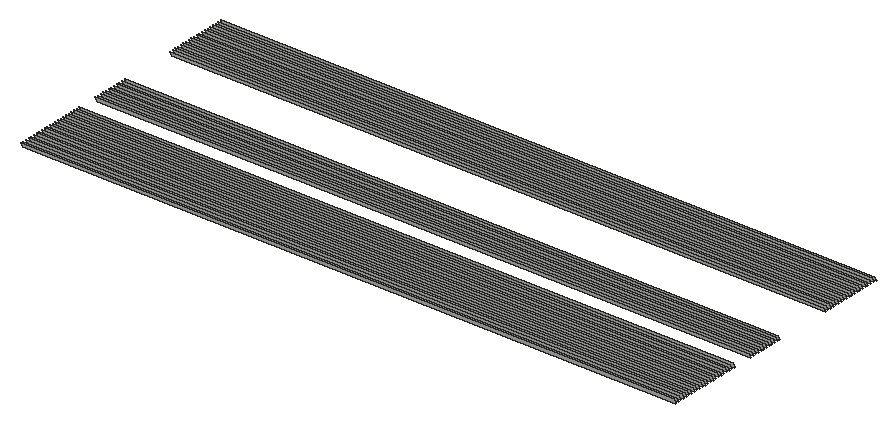
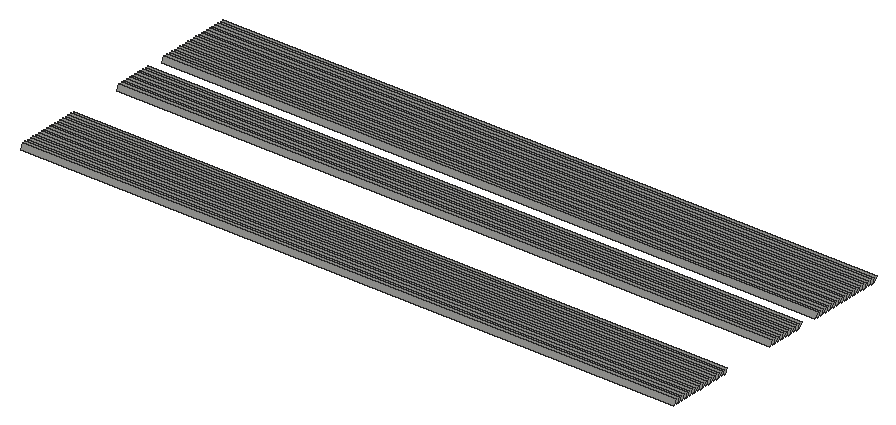
# SketchUp Ruby script. Lengths in inches.
U = 1.inch
M = Sketchup.active_model
def pt(a) = Geom::Point3d.new(a.map { |v| v * U })
def face(e, loops, mat)
  f = e.add_face(loops[0].map { |a| pt(a) })
  loops[1..].each { |l| e.add_face(l.map { |a| pt(a) }).erase! }
  f.material = f.back_material = mat if mat
  f
end
# faces: each face lists its corners as indices into pts; further lists are holes
def faces(e, pts, list, mat = nil) = list.each { |f| face(e, (f[0].is_a?(Array) ? f : [f]).map { |l| l.map { |i| pts[i] } }, mat) }
# xy, xz, yz: faces in a plane at the given z, y or x. An outline is a flat list of corners, or four numbers for a rectangle; further outlines are holes
def ring(l) = l.size == 4 ? [[l[0], l[1]], [l[2], l[1]], [l[2], l[3]], [l[0], l[3]]] : l.each_slice(2).to_a
def flat(e, list, mat, &to3) = list.each { |f| face(e, (f[0].is_a?(Array) ? f : [f]).map { |l| ring(l).map { |u, v| to3.(u, v) } }, mat) }
def xy(e, z, list, mat = nil) = flat(e, list, mat) { |x, y| [x, y, z] }
def xz(e, y, list, mat = nil) = flat(e, list, mat) { |x, z| [x, y, z] }
def yz(e, x, list, mat = nil) = flat(e, list, mat) { |y, z| [x, y, z] }
def lines(e, pts, list) = list.each { |a, b| e.add_line(pt(pts[a]), pt(pts[b])) }
# prism: a flat outline (further loops are holes) pulled along v
def prism(e, loops, v, mat = nil)
  f = face(e, loops, mat); d = Geom::Vector3d.new(v.map { |x| x * U })
  f.pushpull(f.normal.samedirection?(d) ? d.length : -d.length)
end
def box(e, o, s, mat = nil) = prism(e, [[o, [o[0] + s[0], o[1], o[2]], [o[0] + s[0], o[1] + s[1], o[2]], [o[0], o[1] + s[1], o[2]]]], [0, 0, s[2]], mat)
def at(x, y, z, deg = 0) = Geom::Transformation.translation(pt([x, y, z])) * Geom::Transformation.rotation(ORIGIN, Z_AXIS, deg.degrees)
def axes(o, x, y, z) = Geom::Transformation.new([*x, 0, *y, 0, *z, 0, *pt(o).to_a, 1])
def part(name) = M.definitions.add(name)
# library, detail: a bought-in or finely detailed component or shape, given as its bounding box
def library(name, o, s) = part(name).tap { |d| box(d.entities, o, s) }
def detail(e, o, s) = box(e.add_group.entities, o, s)
def put(e, d, t, mat = nil) = e.add_instance(d, t).tap { |i| i.material = mat if mat }
def group(e, t, mat = nil) = e.add_group.tap { |g| g.transformation = t; g.material = mat if mat }.entities
root = M.entities
c1 = part("Group133\#1")
p = [[385.16,-531.55,0],[-385.16,-531.55,0],[-385.16,-534.9375,5.875],[385.16,-534.9375,5.875]]
faces(c1.entities,p,[[0,1,2,3]])
c2 = part("Group134\#1")
p = [[385.16,-527.61,0],[-385.16,-527.61,0],[-385.16,-531,5.875],[385.16,-531,5.875]]
faces(c2.entities,p,[[0,1,2,3]])
c3 = part("Group135\#1")
p = [[-385.16,-527.0625,5.875],[385.16,-527.0625,5.875],[385.16,-523.67,0],[-385.16,-523.67,0]]
faces(c3.entities,p,[[0,1,2,3]])
c4 = part("Group136\#1")
p = [[-385.16,-523.125,5.875],[385.16,-523.125,5.875],[385.16,-519.73,0],[-385.16,-519.73,0]]
faces(c4.entities,p,[[0,1,2,3]])
c5 = part("Group137\#1")
p = [[-385.16,-519.1875,5.875],[385.16,-519.1875,5.875],[385.16,-515.8,0],[-385.16,-515.8,0]]
faces(c5.entities,p,[[0,1,2,3]])
c6 = part("Group138\#1")
p = [[-385.16,-515.25,5.875],[385.16,-515.25,5.875],[385.16,-511.86,0],[-385.16,-511.86,0]]
faces(c6.entities,p,[[0,1,2,3]])
c7 = part("Group139\#1")
p = [[385.16,-507.92,0],[-385.16,-507.92,0],[-385.16,-511.3125,5.875],[385.16,-511.3125,5.875]]
faces(c7.entities,p,[[0,1,2,3]])
c8 = part("Group140\#1")
p = [[385.16,-503.98,0],[-385.16,-503.98,0],[-385.16,-507.375,5.875],[385.16,-507.375,5.875]]
faces(c8.entities,p,[[0,1,2,3]])
c9 = part("Group141\#1")
p = [[-385.16,-503.4375,5.875],[385.16,-503.4375,5.875],[385.16,-500.05,0],[-385.16,-500.05,0]]
faces(c9.entities,p,[[0,1,2,3]])
c10 = part("Group142\#1")
p = [[-385.16,-499.5,5.875],[385.16,-499.5,5.875],[385.16,-496.11,0],[-385.16,-496.11,0]]
faces(c10.entities,p,[[0,1,2,3]])
c11 = part("Group143\#1")
p = [[-385.16,-495.5625,5.875],[385.16,-495.5625,5.875],[385.16,-492.17,0],[-385.16,-492.17,0]]
faces(c11.entities,p,[[0,1,2,3]])
c12 = part("Group144\#1")
p = [[-385.16,-491.625,5.875],[385.16,-491.625,5.875],[385.16,-488.23,0],[-385.16,-488.23,0]]
faces(c12.entities,p,[[0,1,2,3]])
c13 = part("Group145\#1")
p = [[-385.16,-487.6875,5.875],[385.16,-487.6875,5.875],[385.16,-484.3,0],[-385.16,-484.3,0]]
faces(c13.entities,p,[[0,1,2,3]])
c14 = part("Group146\#1")
p = [[385.16,-480.36,0],[-385.16,-480.36,0],[-385.16,-483.75,5.875],[385.16,-483.75,5.875]]
faces(c14.entities,p,[[0,1,2,3]])
c15 = part("Group147\#1")
p = [[-385.16,-479.8125,5.875],[385.16,-479.8125,5.875],[385.16,-476.42,0],[-385.16,-476.42,0]]
faces(c15.entities,p,[[0,1,2,3]])
c16 = part("Group148\#1")
p = [[385.16,-472.48,0],[-385.16,-472.48,0],[-385.16,-475.875,5.875],[385.16,-475.875,5.875]]
faces(c16.entities,p,[[0,1,2,3]])
c17 = part("Group149\#1")
p = [[-385.16,-471.9375,5.875],[385.16,-471.9375,5.875],[385.16,-468.55,0],[-385.16,-468.55,0]]
faces(c17.entities,p,[[0,1,2,3]])
c18 = part("Group150\#1")
p = [[-385.16,-468,5.875],[385.16,-468,5.875],[385.16,-464.61,0],[-385.16,-464.61,0]]
faces(c18.entities,p,[[0,1,2,3]])
c19 = part("Group151\#1")
p = [[-385.16,-464.0625,5.875],[385.16,-464.0625,5.875],[385.16,-460.67,0],[-385.16,-460.67,0]]
faces(c19.entities,p,[[0,1,2,3]])
c20 = part("Group152\#1")
p = [[-385.16,-460.125,5.875],[385.16,-460.125,5.875],[385.16,-456.73,0],[-385.16,-456.73,0]]
faces(c20.entities,p,[[0,1,2,3]])
c21 = part("Group153\#1")
p = [[385.16,-452.8,0],[-385.16,-452.8,0],[-385.16,-456.1875,5.875],[385.16,-456.1875,5.875]]
faces(c21.entities,p,[[0,1,2,3]])
c22 = part("Group154\#1")
p = [[-385.16,-452.25,5.875],[385.16,-452.25,5.875],[385.16,-448.86,0],[-385.16,-448.86,0]]
faces(c22.entities,p,[[0,1,2,3]])
c23 = part("Group155\#1")
p = [[-385.16,-448.3125,5.875],[385.16,-448.3125,5.875],[385.16,-444.92,0],[-385.16,-444.92,0]]
faces(c23.entities,p,[[0,1,2,3]])
c24 = part("Group161\#1")
p = [[-385.16,-424.6875,5.875],[385.16,-424.6875,5.875],[385.16,-421.3,0],[-385.16,-421.3,0]]
faces(c24.entities,p,[[0,1,2,3]])
c25 = part("Group162\#1")
p = [[-385.16,-420.75,5.875],[385.16,-420.75,5.875],[385.16,-417.36,0],[-385.16,-417.36,0]]
faces(c25.entities,p,[[0,1,2,3]])
c26 = part("Group163\#1")
p = [[385.16,-413.42,0],[-385.16,-413.42,0],[-385.16,-416.8125,5.875],[385.16,-416.8125,5.875]]
faces(c26.entities,p,[[0,1,2,3]])
c27 = part("Group164\#1")
p = [[-385.16,-412.875,5.875],[385.16,-412.875,5.875],[385.16,-409.48,0],[-385.16,-409.48,0]]
faces(c27.entities,p,[[0,1,2,3]])
c28 = part("Group165\#1")
p = [[385.16,-405.55,0],[-385.16,-405.55,0],[-385.16,-408.9375,5.875],[385.16,-408.9375,5.875]]
faces(c28.entities,p,[[0,1,2,3]])
c29 = part("Group166\#1")
p = [[385.16,-401.61,0],[-385.16,-401.61,0],[-385.16,-405,5.875],[385.16,-405,5.875]]
faces(c29.entities,p,[[0,1,2,3]])
c30 = part("Group167\#1")
p = [[385.16,-397.67,0],[-385.16,-397.67,0],[-385.16,-401.0625,5.875],[385.16,-401.0625,5.875]]
faces(c30.entities,p,[[0,1,2,3]])
c31 = part("Group168\#1")
p = [[385.16,-393.73,0],[-385.16,-393.73,0],[-385.16,-397.125,5.875],[385.16,-397.125,5.875]]
faces(c31.entities,p,[[0,1,2,3]])
c32 = part("Group169\#1")
p = [[385.16,-389.8,0],[-385.16,-389.8,0],[-385.16,-393.1875,5.875],[385.16,-393.1875,5.875]]
faces(c32.entities,p,[[0,1,2,3]])
c33 = part("Group170\#1")
p = [[-385.16,-389.25,5.875],[385.16,-389.25,5.875],[385.16,-385.86,0],[-385.16,-385.86,0]]
faces(c33.entities,p,[[0,1,2,3]])
c34 = part("Group171\#1")
p = [[385.16,-381.92,0],[-385.16,-381.92,0],[-385.16,-385.3125,5.875],[385.16,-385.3125,5.875]]
faces(c34.entities,p,[[0,1,2,3]])
c35 = part("Group172\#1")
p = [[385.16,-377.98,0],[-385.16,-377.98,0],[-385.16,-381.375,5.875],[385.16,-381.375,5.875]]
faces(c35.entities,p,[[0,1,2,3]])
c36 = part("Group189\#1")
p = [[-385.16,-314.4375,5.875],[385.16,-314.4375,5.875],[385.16,-311.05,0],[-385.16,-311.05,0]]
faces(c36.entities,p,[[0,1,2,3]])
c37 = part("Group190\#1")
p = [[385.16,-307.11,0],[-385.16,-307.11,0],[-385.16,-310.5,5.875],[385.16,-310.5,5.875]]
faces(c37.entities,p,[[0,1,2,3]])
c38 = part("Group191\#1")
p = [[385.16,-303.17,0],[-385.16,-303.17,0],[-385.16,-306.5625,5.875],[385.16,-306.5625,5.875]]
faces(c38.entities,p,[[0,1,2,3]])
c39 = part("Group192\#1")
p = [[-385.16,-302.625,5.875],[385.16,-302.625,5.875],[385.16,-299.23,0],[-385.16,-299.23,0]]
faces(c39.entities,p,[[0,1,2,3]])
c40 = part("Group193\#1")
p = [[-385.16,-298.6875,5.875],[385.16,-298.6875,5.875],[385.16,-295.3,0],[-385.16,-295.3,0]]
faces(c40.entities,p,[[0,1,2,3]])
c41 = part("Group194\#1")
p = [[385.16,-291.36,0],[-385.16,-291.36,0],[-385.16,-294.75,5.875],[385.16,-294.75,5.875]]
faces(c41.entities,p,[[0,1,2,3]])
c42 = part("Group195\#1")
p = [[385.16,-287.42,0],[-385.16,-287.42,0],[-385.16,-290.8125,5.875],[385.16,-290.8125,5.875]]
faces(c42.entities,p,[[0,1,2,3]])
c43 = part("Group196\#1")
p = [[-385.16,-286.875,5.875],[385.16,-286.875,5.875],[385.16,-283.48,0],[-385.16,-283.48,0]]
faces(c43.entities,p,[[0,1,2,3]])
c44 = part("Group197\#1")
p = [[-385.16,-282.9375,5.875],[385.16,-282.9375,5.875],[385.16,-279.55,0],[-385.16,-279.55,0]]
faces(c44.entities,p,[[0,1,2,3]])
c45 = part("Group198\#1")
p = [[385.16,-275.61,0],[-385.16,-275.61,0],[-385.16,-279,5.875],[385.16,-279,5.875]]
faces(c45.entities,p,[[0,1,2,3]])
c46 = part("Group199\#1")
p = [[-385.16,-275.0625,5.875],[385.16,-275.0625,5.875],[385.16,-271.67,0],[-385.16,-271.67,0]]
faces(c46.entities,p,[[0,1,2,3]])
c47 = part("Group200\#1")
p = [[-385.16,-271.125,5.875],[385.16,-271.125,5.875],[385.16,-267.73,0],[-385.16,-267.73,0]]
faces(c47.entities,p,[[0,1,2,3]])
c48 = part("Group201\#1")
p = [[-385.16,-267.1875,5.875],[385.16,-267.1875,5.875],[385.16,-263.8,0],[-385.16,-263.8,0]]
faces(c48.entities,p,[[0,1,2,3]])
c49 = part("Group202\#1")
p = [[-385.16,-263.25,5.875],[385.16,-263.25,5.875],[385.16,-259.86,0],[-385.16,-259.86,0]]
faces(c49.entities,p,[[0,1,2,3]])
c50 = part("Group203\#1")
p = [[-385.16,-259.3125,5.875],[385.16,-259.3125,5.875],[385.16,-255.92,0],[-385.16,-255.92,0]]
faces(c50.entities,p,[[0,1,2,3]])
c51 = part("Group204\#1")
p = [[-385.16,-255.375,5.875],[385.16,-255.375,5.875],[385.16,-251.98,0],[-385.16,-251.98,0]]
faces(c51.entities,p,[[0,1,2,3]])
c52 = part("Group205\#1")
p = [[385.16,-248.05,0],[-385.16,-248.05,0],[-385.16,-251.4375,5.875],[385.16,-251.4375,5.875]]
faces(c52.entities,p,[[0,1,2,3]])
c53 = part("Group206\#1")
p = [[-385.16,-247.5,5.875],[385.16,-247.5,5.875],[385.16,-244.11,0],[-385.16,-244.11,0]]
faces(c53.entities,p,[[0,1,2,3]])
c54 = part("Group207\#1")
p = [[-385.16,-243.5625,5.875],[385.16,-243.5625,5.875],[385.16,-240.17,0],[-385.16,-240.17,0]]
faces(c54.entities,p,[[0,1,2,3]])
c55 = part("Group208\#1")
p = [[385.16,-236.23,0],[-385.16,-236.23,0],[-385.16,-239.625,5.875],[385.16,-239.625,5.875]]
faces(c55.entities,p,[[0,1,2,3]])
put(root,c1,at(1937.93,1232.46,154.625))
put(root,c2,at(1937.93,1232.46,154.625))
put(root,c3,at(1937.93,1232.46,154.625))
put(root,c4,at(1937.93,1232.46,154.625))
put(root,c5,at(1937.93,1232.46,154.625))
put(root,c6,at(1937.93,1232.46,154.625))
put(root,c7,at(1937.93,1232.46,154.625))
put(root,c8,at(1937.93,1232.46,154.625))
put(root,c9,at(1937.93,1232.46,154.625))
put(root,c10,at(1937.93,1232.46,154.625))
put(root,c11,at(1937.93,1232.46,154.625))
put(root,c12,at(1937.93,1232.46,154.625))
put(root,c13,at(1937.93,1232.46,154.625))
put(root,c14,at(1937.93,1232.46,154.625))
put(root,c15,at(1937.93,1232.46,154.625))
put(root,c16,at(1937.93,1232.46,154.625))
put(root,c17,at(1937.93,1232.46,154.625))
put(root,c18,at(1937.93,1232.46,154.625))
put(root,c19,at(1937.93,1232.46,154.625))
put(root,c20,at(1937.93,1232.46,154.625))
put(root,c21,at(1937.93,1232.46,154.625))
put(root,c22,at(1937.93,1232.46,154.625))
put(root,c23,at(1937.93,1232.46,154.625))
put(root,c24,at(1937.93,1232.46,154.625))
put(root,c25,at(1937.93,1232.46,154.625))
put(root,c26,at(1937.93,1232.46,154.625))
put(root,c27,at(1937.93,1232.46,154.625))
put(root,c28,at(1937.93,1232.46,154.625))
put(root,c29,at(1937.93,1232.46,154.625))
put(root,c30,at(1937.93,1232.46,154.625))
put(root,c31,at(1937.93,1232.46,154.625))
put(root,c32,at(1937.93,1232.46,154.625))
put(root,c33,at(1937.93,1232.46,154.625))
put(root,c34,at(1937.93,1232.46,154.625))
put(root,c35,at(1937.93,1232.46,154.625))
put(root,c36,at(1937.93,1232.46,154.625))
put(root,c37,at(1937.93,1232.46,154.625))
put(root,c38,at(1937.93,1232.46,154.625))
put(root,c39,at(1937.93,1232.46,154.625))
put(root,c40,at(1937.93,1232.46,154.625))
put(root,c41,at(1937.93,1232.46,154.625))
put(root,c42,at(1937.93,1232.46,154.625))
put(root,c43,at(1937.93,1232.46,154.625))
put(root,c44,at(1937.93,1232.46,154.625))
put(root,c45,at(1937.93,1232.46,154.625))
put(root,c46,at(1937.93,1232.46,154.625))
put(root,c47,at(1937.93,1232.46,154.625))
put(root,c48,at(1937.93,1232.46,154.625))
put(root,c49,at(1937.93,1232.46,154.625))
put(root,c50,at(1937.93,1232.46,154.625))
put(root,c51,at(1937.93,1232.46,154.625))
put(root,c52,at(1937.93,1232.46,154.625))
put(root,c53,at(1937.93,1232.46,154.625))
put(root,c54,at(1937.93,1232.46,154.625))
put(root,c55,at(1937.93,1232.46,154.625))
